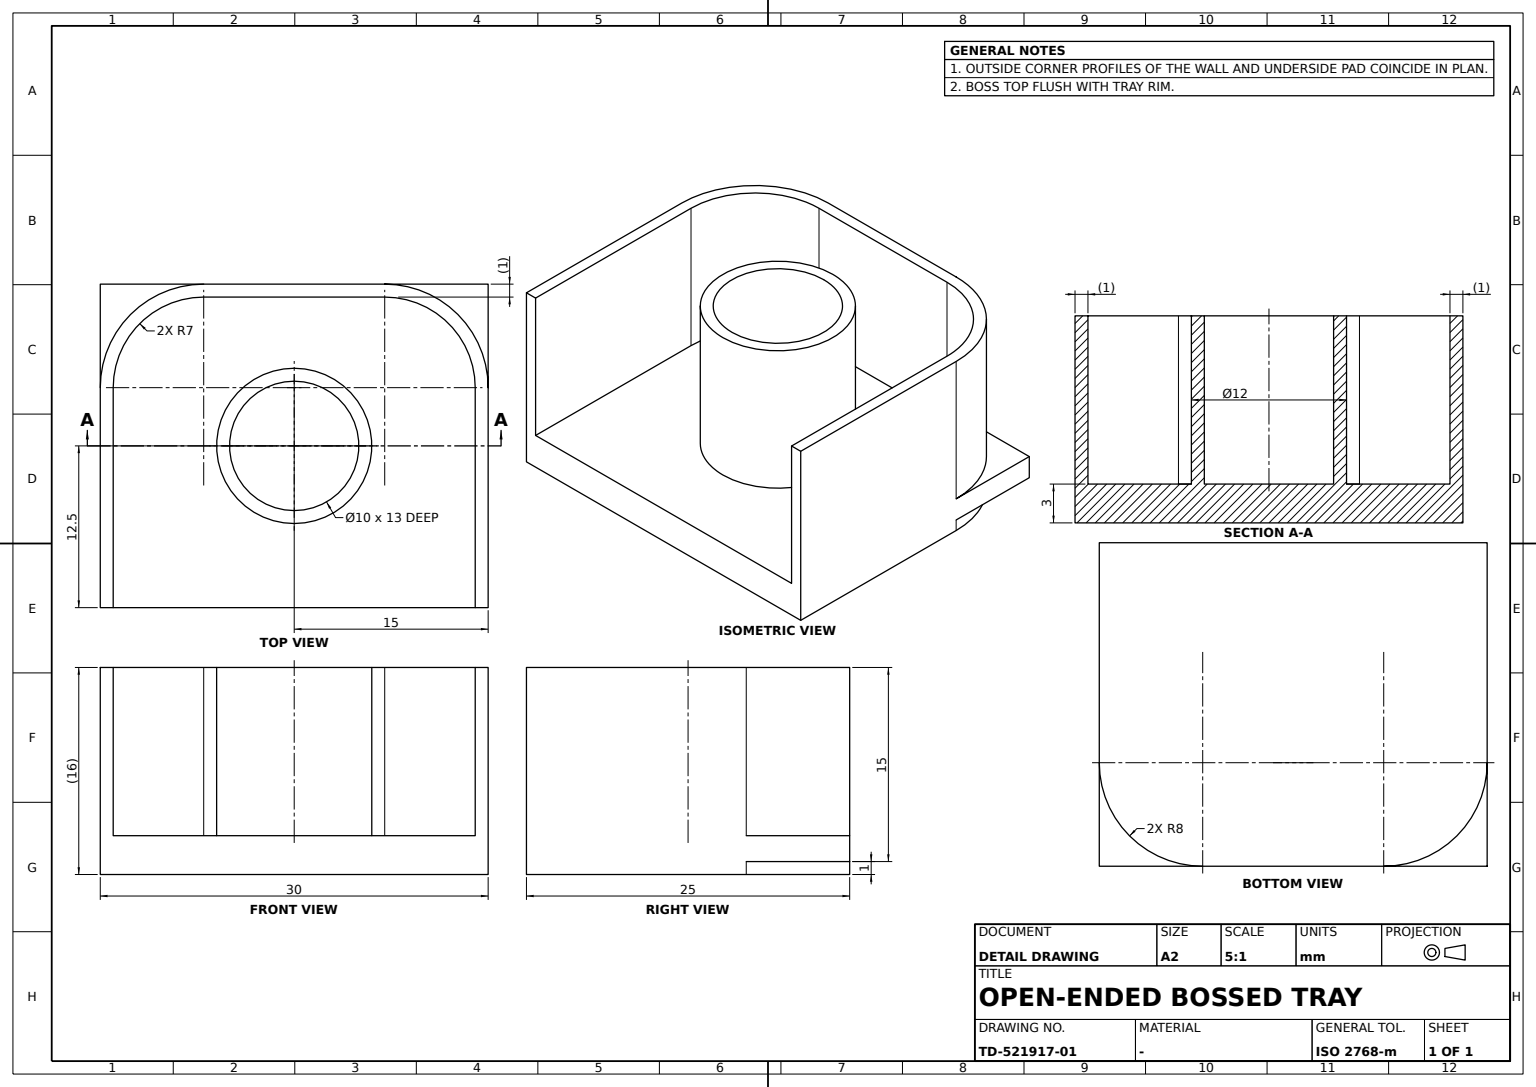
ISO-10303-21;
HEADER;
FILE_DESCRIPTION((''),'2;1');
FILE_NAME('','',(''),(''),'','','');
FILE_SCHEMA(('AUTOMOTIVE_DESIGN'));
ENDSEC;
DATA;
#1=APPLICATION_CONTEXT('');
#2=PRODUCT_CONTEXT('',#1,'mechanical');
#3=PRODUCT('','','',(#2));
#4=PRODUCT_DEFINITION_FORMATION('','',#3);
#5=PRODUCT_DEFINITION_CONTEXT('',#1,'design');
#6=PRODUCT_DEFINITION('','',#4,#5);
#7=PRODUCT_DEFINITION_SHAPE('','',#6);
#8=(LENGTH_UNIT()NAMED_UNIT(*)SI_UNIT(.MILLI.,.METRE.));
#9=(NAMED_UNIT(*)PLANE_ANGLE_UNIT()SI_UNIT($,.RADIAN.));
#10=(NAMED_UNIT(*)SI_UNIT($,.STERADIAN.)SOLID_ANGLE_UNIT());
#11=UNCERTAINTY_MEASURE_WITH_UNIT(LENGTH_MEASURE(1.E-05),#8,'distance_accuracy_value','');
#12=(GEOMETRIC_REPRESENTATION_CONTEXT(3)GLOBAL_UNCERTAINTY_ASSIGNED_CONTEXT((#11))GLOBAL_UNIT_ASSIGNED_CONTEXT((#8,#9,#10))REPRESENTATION_CONTEXT('',''));
#13=CARTESIAN_POINT('',(4.5,14.,3.));
#14=VERTEX_POINT('',#13);
#15=CARTESIAN_POINT('',(4.5,14.,16.));
#16=VERTEX_POINT('',#15);
#17=CARTESIAN_POINT('',(4.5,14.,9.5));
#18=DIRECTION('',(0.,0.,1.));
#19=VECTOR('',#18,1000.);
#20=LINE('',#17,#19);
#21=EDGE_CURVE('',#14,#16,#20,.T.);
#22=ORIENTED_EDGE('',*,*,#21,.F.);
#23=CARTESIAN_POINT('',(11.5,7.,3.));
#24=VERTEX_POINT('',#23);
#25=CARTESIAN_POINT('',(4.5,7.,3.));
#26=DIRECTION('',(1.,0.,0.));
#27=AXIS2_PLACEMENT_3D('',#25,#18,#26);
#28=CIRCLE('',#27,7.);
#29=EDGE_CURVE('',#24,#14,#28,.T.);
#30=ORIENTED_EDGE('',*,*,#29,.F.);
#31=CARTESIAN_POINT('',(11.5,7.,16.));
#32=VERTEX_POINT('',#31);
#33=CARTESIAN_POINT('',(11.5,7.,8.5));
#34=LINE('',#33,#19);
#35=EDGE_CURVE('',#24,#32,#34,.T.);
#36=ORIENTED_EDGE('',*,*,#35,.T.);
#37=CARTESIAN_POINT('',(4.5,7.,16.));
#38=DIRECTION('',(0.,0.,-1.));
#39=AXIS2_PLACEMENT_3D('',#37,#38,#26);
#40=CIRCLE('',#39,7.);
#41=EDGE_CURVE('',#16,#32,#40,.T.);
#42=ORIENTED_EDGE('',*,*,#41,.F.);
#43=EDGE_LOOP('',(#22,#30,#36,#42));
#44=FACE_OUTER_BOUND('',#43,.T.);
#45=CARTESIAN_POINT('',(4.5,7.,8.5));
#46=AXIS2_PLACEMENT_3D('',#45,#38,#26);
#47=CYLINDRICAL_SURFACE('',#46,7.);
#48=ADVANCED_FACE('',(#44),#47,.F.);
#49=CARTESIAN_POINT('',(-5.,0.,3.));
#50=VERTEX_POINT('',#49);
#51=CARTESIAN_POINT('',(5.,0.,3.));
#52=VERTEX_POINT('',#51);
#53=CARTESIAN_POINT('',(0.,0.,3.));
#54=AXIS2_PLACEMENT_3D('',#53,#18,#26);
#55=CIRCLE('',#54,5.);
#56=EDGE_CURVE('',#50,#52,#55,.T.);
#57=ORIENTED_EDGE('',*,*,#56,.F.);
#58=CARTESIAN_POINT('',(-5.,0.,16.));
#59=VERTEX_POINT('',#58);
#60=CARTESIAN_POINT('',(-5.,0.,8.5));
#61=LINE('',#60,#19);
#62=EDGE_CURVE('',#50,#59,#61,.T.);
#63=ORIENTED_EDGE('',*,*,#62,.T.);
#64=CARTESIAN_POINT('',(5.,0.,16.));
#65=VERTEX_POINT('',#64);
#66=CARTESIAN_POINT('',(0.,0.,16.));
#67=AXIS2_PLACEMENT_3D('',#66,#18,#26);
#68=CIRCLE('',#67,5.);
#69=EDGE_CURVE('',#59,#65,#68,.T.);
#70=ORIENTED_EDGE('',*,*,#69,.T.);
#71=CARTESIAN_POINT('',(5.,0.,8.5));
#72=LINE('',#71,#19);
#73=EDGE_CURVE('',#52,#65,#72,.T.);
#74=ORIENTED_EDGE('',*,*,#73,.F.);
#75=EDGE_LOOP('',(#57,#63,#70,#74));
#76=FACE_OUTER_BOUND('',#75,.T.);
#77=CARTESIAN_POINT('',(0.,0.,8.5));
#78=AXIS2_PLACEMENT_3D('',#77,#38,#26);
#79=CYLINDRICAL_SURFACE('',#78,5.);
#80=ADVANCED_FACE('',(#76),#79,.F.);
#81=CARTESIAN_POINT('',(12.5,15.,3.));
#82=VERTEX_POINT('',#81);
#83=CARTESIAN_POINT('',(4.5,15.,3.));
#84=VERTEX_POINT('',#83);
#85=CARTESIAN_POINT('',(8.5,15.,3.));
#86=DIRECTION('',(-1.,0.,0.));
#87=VECTOR('',#86,1000.);
#88=LINE('',#85,#87);
#89=EDGE_CURVE('',#82,#84,#88,.T.);
#90=ORIENTED_EDGE('',*,*,#89,.T.);
#91=CARTESIAN_POINT('',(12.5,7.,3.));
#92=VERTEX_POINT('',#91);
#93=CIRCLE('',#27,8.);
#94=EDGE_CURVE('',#92,#84,#93,.T.);
#95=ORIENTED_EDGE('',*,*,#94,.F.);
#96=CARTESIAN_POINT('',(12.5,11.,3.));
#97=DIRECTION('',(0.,1.,0.));
#98=VECTOR('',#97,1000.);
#99=LINE('',#96,#98);
#100=EDGE_CURVE('',#92,#82,#99,.T.);
#101=ORIENTED_EDGE('',*,*,#100,.T.);
#102=EDGE_LOOP('',(#90,#95,#101));
#103=FACE_OUTER_BOUND('',#102,.T.);
#104=PLANE('',#54);
#105=ADVANCED_FACE('',(#103),#104,.T.);
#106=CARTESIAN_POINT('',(4.5,-15.,16.));
#107=VERTEX_POINT('',#106);
#108=CARTESIAN_POINT('',(12.5,-7.,16.));
#109=VERTEX_POINT('',#108);
#110=CARTESIAN_POINT('',(4.5,-7.,16.));
#111=AXIS2_PLACEMENT_3D('',#110,#18,#26);
#112=CIRCLE('',#111,8.);
#113=EDGE_CURVE('',#107,#109,#112,.T.);
#114=ORIENTED_EDGE('',*,*,#113,.T.);
#115=CARTESIAN_POINT('',(12.5,7.,16.));
#116=VERTEX_POINT('',#115);
#117=CARTESIAN_POINT('',(12.5,0.,16.));
#118=LINE('',#117,#98);
#119=EDGE_CURVE('',#109,#116,#118,.T.);
#120=ORIENTED_EDGE('',*,*,#119,.T.);
#121=CARTESIAN_POINT('',(4.5,15.,16.));
#122=VERTEX_POINT('',#121);
#123=AXIS2_PLACEMENT_3D('',#37,#18,#26);
#124=CIRCLE('',#123,8.);
#125=EDGE_CURVE('',#116,#122,#124,.T.);
#126=ORIENTED_EDGE('',*,*,#125,.T.);
#127=CARTESIAN_POINT('',(-12.5,15.,16.));
#128=VERTEX_POINT('',#127);
#129=CARTESIAN_POINT('',(-4.,15.,16.));
#130=LINE('',#129,#87);
#131=EDGE_CURVE('',#122,#128,#130,.T.);
#132=ORIENTED_EDGE('',*,*,#131,.T.);
#133=CARTESIAN_POINT('',(-12.5,14.,16.));
#134=VERTEX_POINT('',#133);
#135=CARTESIAN_POINT('',(-12.5,14.5,16.));
#136=DIRECTION('',(0.,-1.,0.));
#137=VECTOR('',#136,1000.);
#138=LINE('',#135,#137);
#139=EDGE_CURVE('',#128,#134,#138,.T.);
#140=ORIENTED_EDGE('',*,*,#139,.T.);
#141=CARTESIAN_POINT('',(-4.,14.,16.));
#142=VECTOR('',#26,1000.);
#143=LINE('',#141,#142);
#144=EDGE_CURVE('',#134,#16,#143,.T.);
#145=ORIENTED_EDGE('',*,*,#144,.T.);
#146=ORIENTED_EDGE('',*,*,#41,.T.);
#147=CARTESIAN_POINT('',(11.5,-7.,16.));
#148=VERTEX_POINT('',#147);
#149=CARTESIAN_POINT('',(11.5,0.,16.));
#150=LINE('',#149,#137);
#151=EDGE_CURVE('',#32,#148,#150,.T.);
#152=ORIENTED_EDGE('',*,*,#151,.T.);
#153=CARTESIAN_POINT('',(4.5,-14.,16.));
#154=VERTEX_POINT('',#153);
#155=AXIS2_PLACEMENT_3D('',#110,#38,#26);
#156=CIRCLE('',#155,7.);
#157=EDGE_CURVE('',#148,#154,#156,.T.);
#158=ORIENTED_EDGE('',*,*,#157,.T.);
#159=CARTESIAN_POINT('',(-12.5,-14.,16.));
#160=VERTEX_POINT('',#159);
#161=CARTESIAN_POINT('',(-4.,-14.,16.));
#162=LINE('',#161,#87);
#163=EDGE_CURVE('',#154,#160,#162,.T.);
#164=ORIENTED_EDGE('',*,*,#163,.T.);
#165=CARTESIAN_POINT('',(-12.5,-15.,16.));
#166=VERTEX_POINT('',#165);
#167=CARTESIAN_POINT('',(-12.5,-14.5,16.));
#168=LINE('',#167,#137);
#169=EDGE_CURVE('',#160,#166,#168,.T.);
#170=ORIENTED_EDGE('',*,*,#169,.T.);
#171=CARTESIAN_POINT('',(-4.,-15.,16.));
#172=LINE('',#171,#142);
#173=EDGE_CURVE('',#166,#107,#172,.T.);
#174=ORIENTED_EDGE('',*,*,#173,.T.);
#175=EDGE_LOOP('',(#114,#120,#126,#132,#140,#145,#146,#152,#158,#164,#170,#174));
#176=FACE_OUTER_BOUND('',#175,.T.);
#177=PLANE('',#67);
#178=ADVANCED_FACE('',(#176),#177,.T.);
#179=CARTESIAN_POINT('',(-6.,0.,16.));
#180=VERTEX_POINT('',#179);
#181=CARTESIAN_POINT('',(6.,0.,16.));
#182=VERTEX_POINT('',#181);
#183=CIRCLE('',#67,6.);
#184=EDGE_CURVE('',#180,#182,#183,.T.);
#185=ORIENTED_EDGE('',*,*,#184,.T.);
#186=EDGE_CURVE('',#182,#180,#183,.T.);
#187=ORIENTED_EDGE('',*,*,#186,.T.);
#188=EDGE_LOOP('',(#185,#187));
#189=FACE_OUTER_BOUND('',#188,.T.);
#190=EDGE_CURVE('',#65,#59,#68,.T.);
#191=ORIENTED_EDGE('',*,*,#190,.F.);
#192=ORIENTED_EDGE('',*,*,#69,.F.);
#193=EDGE_LOOP('',(#191,#192));
#194=FACE_BOUND('',#193,.T.);
#195=ADVANCED_FACE('',(#189,#194),#177,.T.);
#196=CARTESIAN_POINT('',(11.5,-7.,3.));
#197=VERTEX_POINT('',#196);
#198=CARTESIAN_POINT('',(11.5,-7.,9.5));
#199=LINE('',#198,#19);
#200=EDGE_CURVE('',#197,#148,#199,.T.);
#201=ORIENTED_EDGE('',*,*,#200,.T.);
#202=ORIENTED_EDGE('',*,*,#151,.F.);
#203=ORIENTED_EDGE('',*,*,#35,.F.);
#204=CARTESIAN_POINT('',(11.5,0.,3.));
#205=LINE('',#204,#137);
#206=EDGE_CURVE('',#24,#197,#205,.T.);
#207=ORIENTED_EDGE('',*,*,#206,.T.);
#208=EDGE_LOOP('',(#201,#202,#203,#207));
#209=FACE_OUTER_BOUND('',#208,.T.);
#210=CARTESIAN_POINT('',(11.5,7.,1.));
#211=AXIS2_PLACEMENT_3D('',#210,#86,#136);
#212=PLANE('',#211);
#213=ADVANCED_FACE('',(#209),#212,.T.);
#214=ORIENTED_EDGE('',*,*,#125,.F.);
#215=CARTESIAN_POINT('',(12.5,7.,9.5));
#216=LINE('',#215,#19);
#217=EDGE_CURVE('',#92,#116,#216,.T.);
#218=ORIENTED_EDGE('',*,*,#217,.F.);
#219=ORIENTED_EDGE('',*,*,#94,.T.);
#220=CARTESIAN_POINT('',(4.5,15.,9.5));
#221=LINE('',#220,#19);
#222=EDGE_CURVE('',#84,#122,#221,.T.);
#223=ORIENTED_EDGE('',*,*,#222,.T.);
#224=EDGE_LOOP('',(#214,#218,#219,#223));
#225=FACE_OUTER_BOUND('',#224,.T.);
#226=CYLINDRICAL_SURFACE('',#46,8.);
#227=ADVANCED_FACE('',(#225),#226,.T.);
#228=CARTESIAN_POINT('',(4.5,-15.,3.));
#229=VERTEX_POINT('',#228);
#230=CARTESIAN_POINT('',(12.5,-7.,3.));
#231=VERTEX_POINT('',#230);
#232=CARTESIAN_POINT('',(4.5,-7.,3.));
#233=AXIS2_PLACEMENT_3D('',#232,#18,#26);
#234=CIRCLE('',#233,8.);
#235=EDGE_CURVE('',#229,#231,#234,.T.);
#236=ORIENTED_EDGE('',*,*,#235,.T.);
#237=CARTESIAN_POINT('',(12.5,-7.,9.5));
#238=LINE('',#237,#19);
#239=EDGE_CURVE('',#231,#109,#238,.T.);
#240=ORIENTED_EDGE('',*,*,#239,.T.);
#241=ORIENTED_EDGE('',*,*,#113,.F.);
#242=CARTESIAN_POINT('',(4.5,-15.,9.5));
#243=LINE('',#242,#19);
#244=EDGE_CURVE('',#229,#107,#243,.T.);
#245=ORIENTED_EDGE('',*,*,#244,.F.);
#246=EDGE_LOOP('',(#236,#240,#241,#245));
#247=FACE_OUTER_BOUND('',#246,.T.);
#248=CARTESIAN_POINT('',(4.5,-7.,0.5));
#249=AXIS2_PLACEMENT_3D('',#248,#38,#26);
#250=CYLINDRICAL_SURFACE('',#249,8.);
#251=ADVANCED_FACE('',(#247),#250,.T.);
#252=ORIENTED_EDGE('',*,*,#235,.F.);
#253=CARTESIAN_POINT('',(12.5,-15.,3.));
#254=VERTEX_POINT('',#253);
#255=CARTESIAN_POINT('',(8.5,-15.,3.));
#256=LINE('',#255,#142);
#257=EDGE_CURVE('',#229,#254,#256,.T.);
#258=ORIENTED_EDGE('',*,*,#257,.T.);
#259=CARTESIAN_POINT('',(12.5,-11.,3.));
#260=LINE('',#259,#98);
#261=EDGE_CURVE('',#254,#231,#260,.T.);
#262=ORIENTED_EDGE('',*,*,#261,.T.);
#263=EDGE_LOOP('',(#252,#258,#262));
#264=FACE_OUTER_BOUND('',#263,.T.);
#265=ADVANCED_FACE('',(#264),#104,.T.);
#266=CARTESIAN_POINT('',(4.5,-15.,1.));
#267=VERTEX_POINT('',#266);
#268=CARTESIAN_POINT('',(12.5,-15.,1.));
#269=VERTEX_POINT('',#268);
#270=CARTESIAN_POINT('',(8.5,-15.,1.));
#271=LINE('',#270,#142);
#272=EDGE_CURVE('',#267,#269,#271,.T.);
#273=ORIENTED_EDGE('',*,*,#272,.F.);
#274=CARTESIAN_POINT('',(12.5,-7.,1.));
#275=VERTEX_POINT('',#274);
#276=CARTESIAN_POINT('',(4.5,-7.,1.));
#277=AXIS2_PLACEMENT_3D('',#276,#18,#26);
#278=CIRCLE('',#277,8.);
#279=EDGE_CURVE('',#267,#275,#278,.T.);
#280=ORIENTED_EDGE('',*,*,#279,.T.);
#281=CARTESIAN_POINT('',(12.5,-11.,1.));
#282=LINE('',#281,#98);
#283=EDGE_CURVE('',#269,#275,#282,.T.);
#284=ORIENTED_EDGE('',*,*,#283,.F.);
#285=EDGE_LOOP('',(#273,#280,#284));
#286=FACE_OUTER_BOUND('',#285,.T.);
#287=CARTESIAN_POINT('',(0.,0.,1.));
#288=AXIS2_PLACEMENT_3D('',#287,#18,#26);
#289=PLANE('',#288);
#290=ADVANCED_FACE('',(#286),#289,.F.);
#291=CARTESIAN_POINT('',(4.5,15.,0.));
#292=VERTEX_POINT('',#291);
#293=CARTESIAN_POINT('',(-12.5,15.,0.));
#294=VERTEX_POINT('',#293);
#295=CARTESIAN_POINT('',(-4.,15.,0.));
#296=LINE('',#295,#87);
#297=EDGE_CURVE('',#292,#294,#296,.T.);
#298=ORIENTED_EDGE('',*,*,#297,.T.);
#299=CARTESIAN_POINT('',(-12.5,15.,8.));
#300=LINE('',#299,#19);
#301=EDGE_CURVE('',#294,#128,#300,.T.);
#302=ORIENTED_EDGE('',*,*,#301,.T.);
#303=ORIENTED_EDGE('',*,*,#131,.F.);
#304=ORIENTED_EDGE('',*,*,#222,.F.);
#305=ORIENTED_EDGE('',*,*,#89,.F.);
#306=CARTESIAN_POINT('',(12.5,15.,1.));
#307=VERTEX_POINT('',#306);
#308=CARTESIAN_POINT('',(12.5,15.,2.));
#309=LINE('',#308,#19);
#310=EDGE_CURVE('',#307,#82,#309,.T.);
#311=ORIENTED_EDGE('',*,*,#310,.F.);
#312=CARTESIAN_POINT('',(4.5,15.,1.));
#313=VERTEX_POINT('',#312);
#314=CARTESIAN_POINT('',(8.5,15.,1.));
#315=LINE('',#314,#87);
#316=EDGE_CURVE('',#307,#313,#315,.T.);
#317=ORIENTED_EDGE('',*,*,#316,.T.);
#318=CARTESIAN_POINT('',(4.5,15.,0.5));
#319=LINE('',#318,#19);
#320=EDGE_CURVE('',#292,#313,#319,.T.);
#321=ORIENTED_EDGE('',*,*,#320,.F.);
#322=EDGE_LOOP('',(#298,#302,#303,#304,#305,#311,#317,#321));
#323=FACE_OUTER_BOUND('',#322,.T.);
#324=AXIS2_PLACEMENT_3D('',#293,#136,#26);
#325=PLANE('',#324);
#326=ADVANCED_FACE('',(#323),#325,.F.);
#327=ORIENTED_EDGE('',*,*,#316,.F.);
#328=CARTESIAN_POINT('',(12.5,7.,1.));
#329=VERTEX_POINT('',#328);
#330=CARTESIAN_POINT('',(12.5,11.,1.));
#331=LINE('',#330,#98);
#332=EDGE_CURVE('',#329,#307,#331,.T.);
#333=ORIENTED_EDGE('',*,*,#332,.F.);
#334=CARTESIAN_POINT('',(4.5,7.,1.));
#335=AXIS2_PLACEMENT_3D('',#334,#18,#26);
#336=CIRCLE('',#335,8.);
#337=EDGE_CURVE('',#329,#313,#336,.T.);
#338=ORIENTED_EDGE('',*,*,#337,.T.);
#339=EDGE_LOOP('',(#327,#333,#338));
#340=FACE_OUTER_BOUND('',#339,.T.);
#341=ADVANCED_FACE('',(#340),#289,.F.);
#342=ORIENTED_EDGE('',*,*,#21,.T.);
#343=ORIENTED_EDGE('',*,*,#144,.F.);
#344=CARTESIAN_POINT('',(-12.5,14.,3.));
#345=VERTEX_POINT('',#344);
#346=CARTESIAN_POINT('',(-12.5,14.,9.5));
#347=LINE('',#346,#19);
#348=EDGE_CURVE('',#345,#134,#347,.T.);
#349=ORIENTED_EDGE('',*,*,#348,.F.);
#350=CARTESIAN_POINT('',(-4.,14.,3.));
#351=LINE('',#350,#142);
#352=EDGE_CURVE('',#345,#14,#351,.T.);
#353=ORIENTED_EDGE('',*,*,#352,.T.);
#354=EDGE_LOOP('',(#342,#343,#349,#353));
#355=FACE_OUTER_BOUND('',#354,.T.);
#356=CARTESIAN_POINT('',(4.5,14.,1.));
#357=AXIS2_PLACEMENT_3D('',#356,#97,#86);
#358=PLANE('',#357);
#359=ADVANCED_FACE('',(#355),#358,.F.);
#360=CARTESIAN_POINT('',(-12.5,-14.,3.));
#361=VERTEX_POINT('',#360);
#362=CARTESIAN_POINT('',(-12.5,-14.,9.5));
#363=LINE('',#362,#19);
#364=EDGE_CURVE('',#361,#160,#363,.T.);
#365=ORIENTED_EDGE('',*,*,#364,.T.);
#366=ORIENTED_EDGE('',*,*,#163,.F.);
#367=CARTESIAN_POINT('',(4.5,-14.,3.));
#368=VERTEX_POINT('',#367);
#369=CARTESIAN_POINT('',(4.5,-14.,8.5));
#370=LINE('',#369,#19);
#371=EDGE_CURVE('',#368,#154,#370,.T.);
#372=ORIENTED_EDGE('',*,*,#371,.F.);
#373=CARTESIAN_POINT('',(-4.,-14.,3.));
#374=LINE('',#373,#142);
#375=EDGE_CURVE('',#361,#368,#374,.T.);
#376=ORIENTED_EDGE('',*,*,#375,.F.);
#377=EDGE_LOOP('',(#365,#366,#372,#376));
#378=FACE_OUTER_BOUND('',#377,.T.);
#379=CARTESIAN_POINT('',(4.5,-14.,1.));
#380=AXIS2_PLACEMENT_3D('',#379,#97,#86);
#381=PLANE('',#380);
#382=ADVANCED_FACE('',(#378),#381,.T.);
#383=EDGE_CURVE('',#52,#50,#55,.T.);
#384=ORIENTED_EDGE('',*,*,#383,.T.);
#385=ORIENTED_EDGE('',*,*,#56,.T.);
#386=EDGE_LOOP('',(#384,#385));
#387=FACE_OUTER_BOUND('',#386,.T.);
#388=ADVANCED_FACE('',(#387),#104,.T.);
#389=ORIENTED_EDGE('',*,*,#73,.T.);
#390=ORIENTED_EDGE('',*,*,#190,.T.);
#391=ORIENTED_EDGE('',*,*,#62,.F.);
#392=ORIENTED_EDGE('',*,*,#383,.F.);
#393=EDGE_LOOP('',(#389,#390,#391,#392));
#394=FACE_OUTER_BOUND('',#393,.T.);
#395=ADVANCED_FACE('',(#394),#79,.F.);
#396=ORIENTED_EDGE('',*,*,#244,.T.);
#397=ORIENTED_EDGE('',*,*,#173,.F.);
#398=CARTESIAN_POINT('',(-12.5,-15.,0.));
#399=VERTEX_POINT('',#398);
#400=CARTESIAN_POINT('',(-12.5,-15.,8.));
#401=LINE('',#400,#19);
#402=EDGE_CURVE('',#399,#166,#401,.T.);
#403=ORIENTED_EDGE('',*,*,#402,.F.);
#404=CARTESIAN_POINT('',(4.5,-15.,0.));
#405=VERTEX_POINT('',#404);
#406=CARTESIAN_POINT('',(-4.,-15.,0.));
#407=LINE('',#406,#142);
#408=EDGE_CURVE('',#399,#405,#407,.T.);
#409=ORIENTED_EDGE('',*,*,#408,.T.);
#410=CARTESIAN_POINT('',(4.5,-15.,0.5));
#411=LINE('',#410,#19);
#412=EDGE_CURVE('',#405,#267,#411,.T.);
#413=ORIENTED_EDGE('',*,*,#412,.T.);
#414=ORIENTED_EDGE('',*,*,#272,.T.);
#415=CARTESIAN_POINT('',(12.5,-15.,2.));
#416=LINE('',#415,#19);
#417=EDGE_CURVE('',#269,#254,#416,.T.);
#418=ORIENTED_EDGE('',*,*,#417,.T.);
#419=ORIENTED_EDGE('',*,*,#257,.F.);
#420=EDGE_LOOP('',(#396,#397,#403,#409,#413,#414,#418,#419));
#421=FACE_OUTER_BOUND('',#420,.T.);
#422=CARTESIAN_POINT('',(12.5,-15.,0.));
#423=AXIS2_PLACEMENT_3D('',#422,#97,#86);
#424=PLANE('',#423);
#425=ADVANCED_FACE('',(#421),#424,.F.);
#426=CIRCLE('',#233,7.);
#427=EDGE_CURVE('',#368,#197,#426,.T.);
#428=ORIENTED_EDGE('',*,*,#427,.F.);
#429=ORIENTED_EDGE('',*,*,#371,.T.);
#430=ORIENTED_EDGE('',*,*,#157,.F.);
#431=ORIENTED_EDGE('',*,*,#200,.F.);
#432=EDGE_LOOP('',(#428,#429,#430,#431));
#433=FACE_OUTER_BOUND('',#432,.T.);
#434=CARTESIAN_POINT('',(4.5,-7.,8.5));
#435=AXIS2_PLACEMENT_3D('',#434,#38,#26);
#436=CYLINDRICAL_SURFACE('',#435,7.);
#437=ADVANCED_FACE('',(#433),#436,.F.);
#438=ORIENTED_EDGE('',*,*,#352,.F.);
#439=CARTESIAN_POINT('',(-12.5,0.,3.));
#440=LINE('',#439,#137);
#441=EDGE_CURVE('',#345,#361,#440,.T.);
#442=ORIENTED_EDGE('',*,*,#441,.T.);
#443=ORIENTED_EDGE('',*,*,#375,.T.);
#444=ORIENTED_EDGE('',*,*,#427,.T.);
#445=ORIENTED_EDGE('',*,*,#206,.F.);
#446=ORIENTED_EDGE('',*,*,#29,.T.);
#447=EDGE_LOOP('',(#438,#442,#443,#444,#445,#446));
#448=FACE_OUTER_BOUND('',#447,.T.);
#449=CARTESIAN_POINT('',(6.,0.,3.));
#450=VERTEX_POINT('',#449);
#451=CARTESIAN_POINT('',(-6.,0.,3.));
#452=VERTEX_POINT('',#451);
#453=CIRCLE('',#54,6.);
#454=EDGE_CURVE('',#450,#452,#453,.T.);
#455=ORIENTED_EDGE('',*,*,#454,.F.);
#456=EDGE_CURVE('',#452,#450,#453,.T.);
#457=ORIENTED_EDGE('',*,*,#456,.F.);
#458=EDGE_LOOP('',(#455,#457));
#459=FACE_BOUND('',#458,.T.);
#460=ADVANCED_FACE('',(#448,#459),#104,.T.);
#461=ORIENTED_EDGE('',*,*,#412,.F.);
#462=CARTESIAN_POINT('',(12.5,-7.,0.));
#463=VERTEX_POINT('',#462);
#464=CARTESIAN_POINT('',(4.5,-7.,0.));
#465=AXIS2_PLACEMENT_3D('',#464,#18,#26);
#466=CIRCLE('',#465,8.);
#467=EDGE_CURVE('',#405,#463,#466,.T.);
#468=ORIENTED_EDGE('',*,*,#467,.T.);
#469=CARTESIAN_POINT('',(12.5,-7.,0.5));
#470=LINE('',#469,#19);
#471=EDGE_CURVE('',#463,#275,#470,.T.);
#472=ORIENTED_EDGE('',*,*,#471,.T.);
#473=ORIENTED_EDGE('',*,*,#279,.F.);
#474=EDGE_LOOP('',(#461,#468,#472,#473));
#475=FACE_OUTER_BOUND('',#474,.T.);
#476=ADVANCED_FACE('',(#475),#250,.T.);
#477=ORIENTED_EDGE('',*,*,#467,.F.);
#478=ORIENTED_EDGE('',*,*,#408,.F.);
#479=CARTESIAN_POINT('',(-12.5,0.,0.));
#480=LINE('',#479,#137);
#481=EDGE_CURVE('',#294,#399,#480,.T.);
#482=ORIENTED_EDGE('',*,*,#481,.F.);
#483=ORIENTED_EDGE('',*,*,#297,.F.);
#484=CARTESIAN_POINT('',(12.5,7.,0.));
#485=VERTEX_POINT('',#484);
#486=CARTESIAN_POINT('',(4.5,7.,0.));
#487=AXIS2_PLACEMENT_3D('',#486,#18,#26);
#488=CIRCLE('',#487,8.);
#489=EDGE_CURVE('',#485,#292,#488,.T.);
#490=ORIENTED_EDGE('',*,*,#489,.F.);
#491=CARTESIAN_POINT('',(12.5,0.,0.));
#492=LINE('',#491,#98);
#493=EDGE_CURVE('',#463,#485,#492,.T.);
#494=ORIENTED_EDGE('',*,*,#493,.F.);
#495=EDGE_LOOP('',(#477,#478,#482,#483,#490,#494));
#496=FACE_OUTER_BOUND('',#495,.T.);
#497=CARTESIAN_POINT('',(0.,0.,0.));
#498=AXIS2_PLACEMENT_3D('',#497,#18,#26);
#499=PLANE('',#498);
#500=ADVANCED_FACE('',(#496),#499,.F.);
#501=ORIENTED_EDGE('',*,*,#456,.T.);
#502=CARTESIAN_POINT('',(6.,0.,8.5));
#503=LINE('',#502,#19);
#504=EDGE_CURVE('',#450,#182,#503,.T.);
#505=ORIENTED_EDGE('',*,*,#504,.T.);
#506=ORIENTED_EDGE('',*,*,#184,.F.);
#507=CARTESIAN_POINT('',(-6.,0.,8.5));
#508=LINE('',#507,#19);
#509=EDGE_CURVE('',#452,#180,#508,.T.);
#510=ORIENTED_EDGE('',*,*,#509,.F.);
#511=EDGE_LOOP('',(#501,#505,#506,#510));
#512=FACE_OUTER_BOUND('',#511,.T.);
#513=CYLINDRICAL_SURFACE('',#78,6.);
#514=ADVANCED_FACE('',(#512),#513,.T.);
#515=ORIENTED_EDGE('',*,*,#489,.T.);
#516=ORIENTED_EDGE('',*,*,#320,.T.);
#517=ORIENTED_EDGE('',*,*,#337,.F.);
#518=CARTESIAN_POINT('',(12.5,7.,0.5));
#519=LINE('',#518,#19);
#520=EDGE_CURVE('',#485,#329,#519,.T.);
#521=ORIENTED_EDGE('',*,*,#520,.F.);
#522=EDGE_LOOP('',(#515,#516,#517,#521));
#523=FACE_OUTER_BOUND('',#522,.T.);
#524=ADVANCED_FACE('',(#523),#226,.T.);
#525=ORIENTED_EDGE('',*,*,#217,.T.);
#526=ORIENTED_EDGE('',*,*,#119,.F.);
#527=ORIENTED_EDGE('',*,*,#239,.F.);
#528=ORIENTED_EDGE('',*,*,#261,.F.);
#529=ORIENTED_EDGE('',*,*,#417,.F.);
#530=ORIENTED_EDGE('',*,*,#283,.T.);
#531=ORIENTED_EDGE('',*,*,#471,.F.);
#532=ORIENTED_EDGE('',*,*,#493,.T.);
#533=ORIENTED_EDGE('',*,*,#520,.T.);
#534=ORIENTED_EDGE('',*,*,#332,.T.);
#535=ORIENTED_EDGE('',*,*,#310,.T.);
#536=ORIENTED_EDGE('',*,*,#100,.F.);
#537=EDGE_LOOP('',(#525,#526,#527,#528,#529,#530,#531,#532,#533,#534,#535,#536));
#538=FACE_OUTER_BOUND('',#537,.T.);
#539=CARTESIAN_POINT('',(12.5,15.,0.));
#540=AXIS2_PLACEMENT_3D('',#539,#86,#136);
#541=PLANE('',#540);
#542=ADVANCED_FACE('',(#538),#541,.F.);
#543=ORIENTED_EDGE('',*,*,#481,.T.);
#544=ORIENTED_EDGE('',*,*,#402,.T.);
#545=ORIENTED_EDGE('',*,*,#169,.F.);
#546=ORIENTED_EDGE('',*,*,#364,.F.);
#547=ORIENTED_EDGE('',*,*,#441,.F.);
#548=ORIENTED_EDGE('',*,*,#348,.T.);
#549=ORIENTED_EDGE('',*,*,#139,.F.);
#550=ORIENTED_EDGE('',*,*,#301,.F.);
#551=EDGE_LOOP('',(#543,#544,#545,#546,#547,#548,#549,#550));
#552=FACE_OUTER_BOUND('',#551,.T.);
#553=AXIS2_PLACEMENT_3D('',#398,#26,#97);
#554=PLANE('',#553);
#555=ADVANCED_FACE('',(#552),#554,.F.);
#556=ORIENTED_EDGE('',*,*,#186,.F.);
#557=ORIENTED_EDGE('',*,*,#504,.F.);
#558=ORIENTED_EDGE('',*,*,#454,.T.);
#559=ORIENTED_EDGE('',*,*,#509,.T.);
#560=EDGE_LOOP('',(#556,#557,#558,#559));
#561=FACE_OUTER_BOUND('',#560,.T.);
#562=ADVANCED_FACE('',(#561),#513,.T.);
#563=CLOSED_SHELL('',(#48,#80,#105,#178,#195,#213,#227,#251,#265,#290,#326,#341,#359,#382,#388,#395,#425,#437,#460,#476,#500,#514,#524,#542,#555,#562));
#564=MANIFOLD_SOLID_BREP('',#563);
#565=ADVANCED_BREP_SHAPE_REPRESENTATION('',(#564),#12);
#566=SHAPE_DEFINITION_REPRESENTATION(#7,#565);
ENDSEC;
END-ISO-10303-21;
